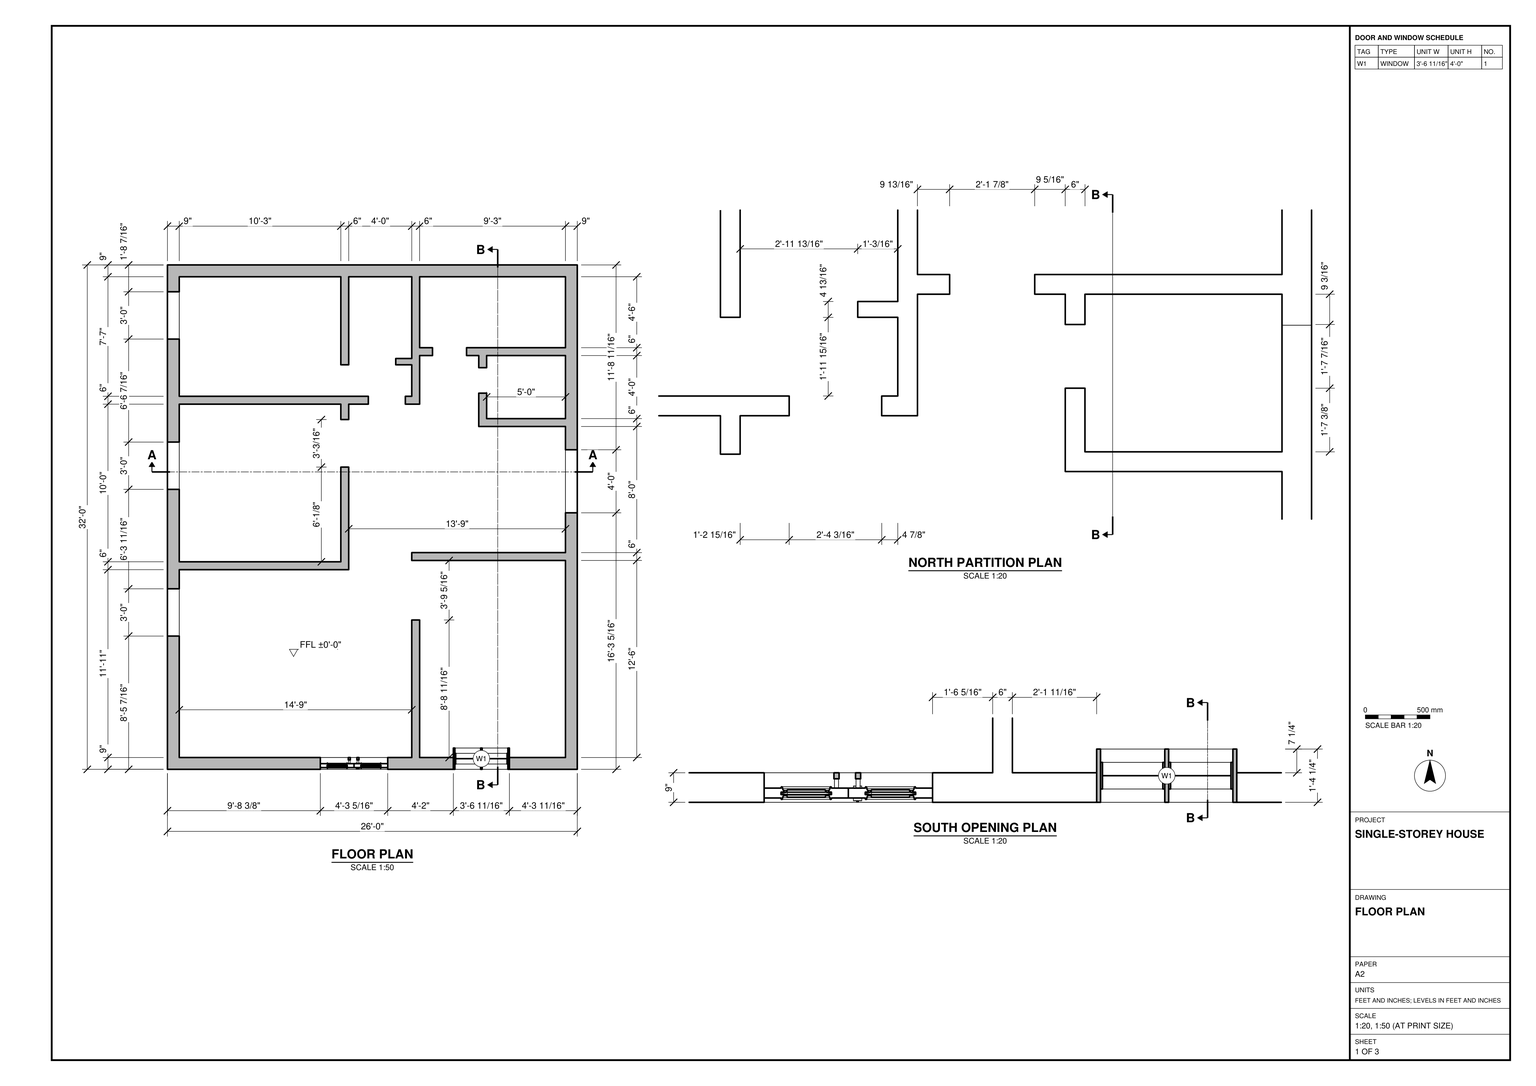
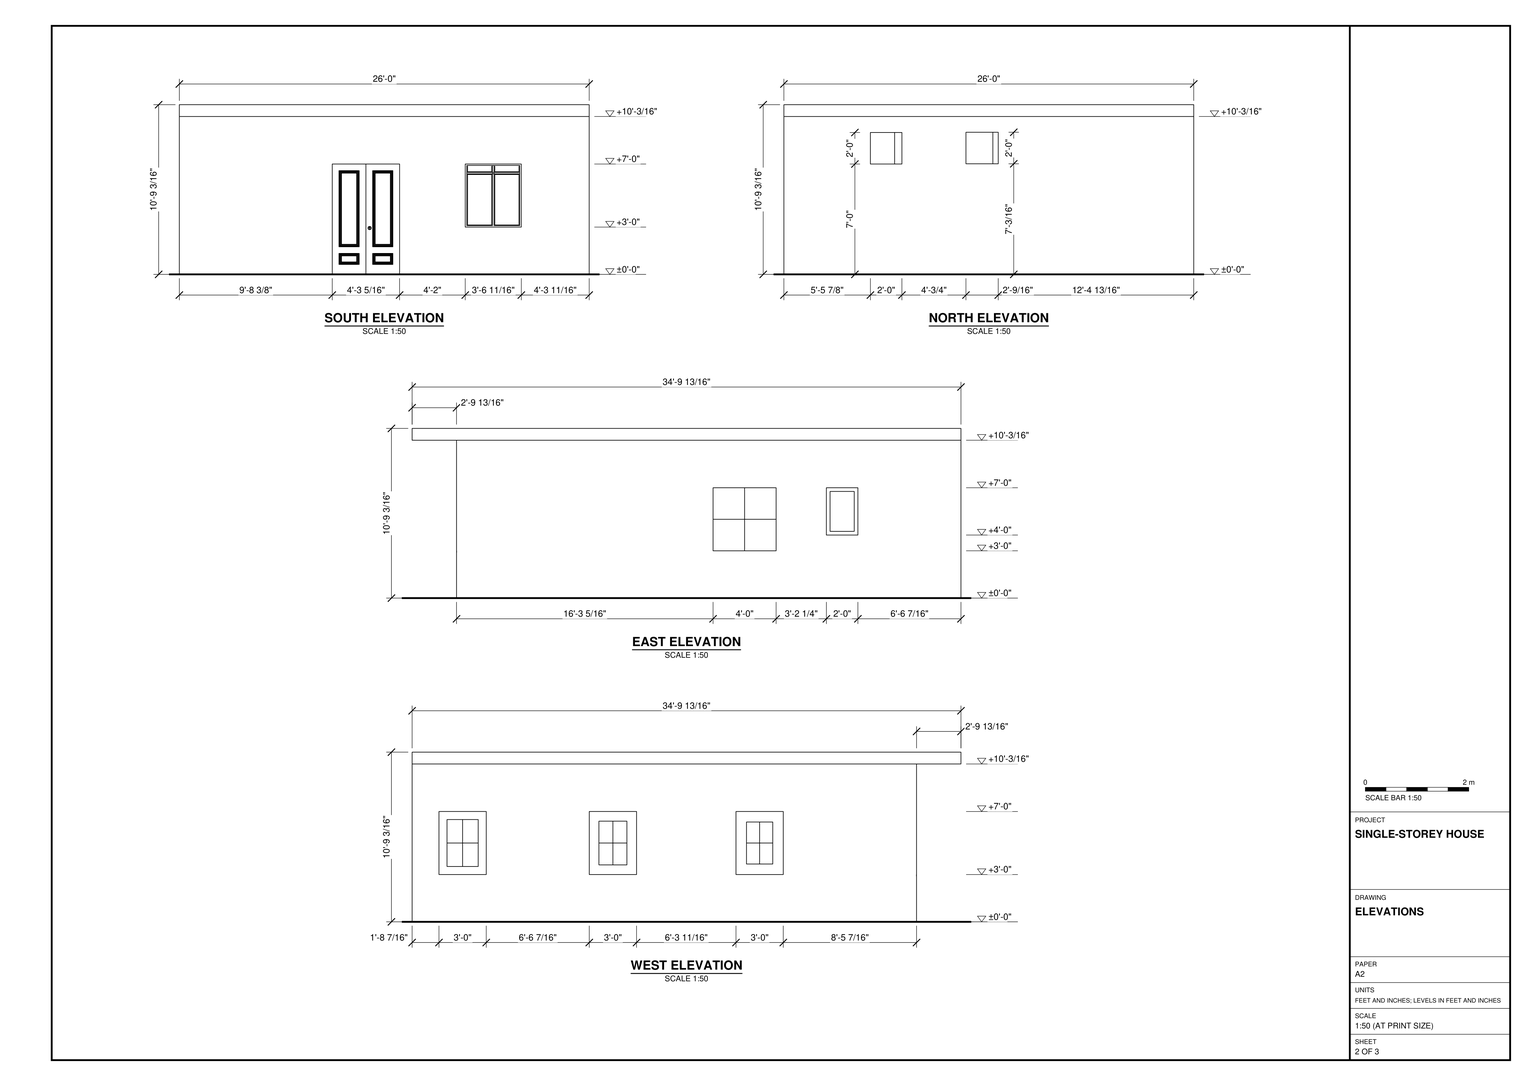
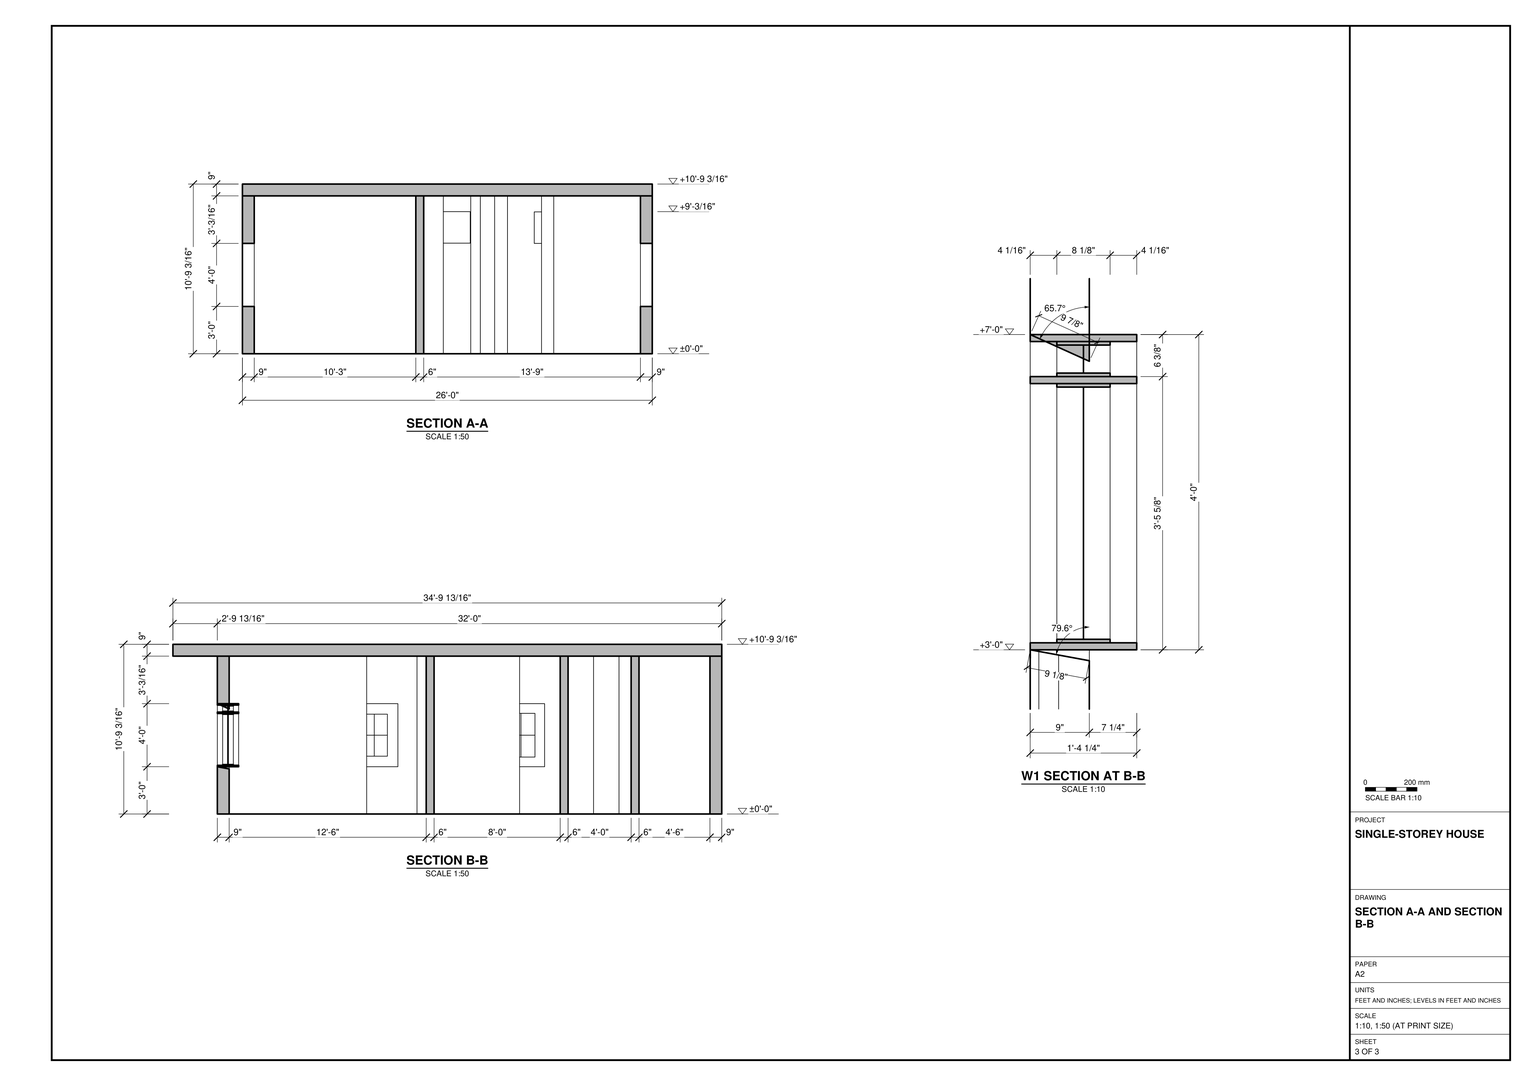
Build the single-storey house in SketchUp from task_files/diagram_01.pdf. Work in feet and inches. Set the finished ground floor at ±0'-0". The overall model is 26'-0" wide, 34'-9 13/16" deep and 10'-9 3/16" high. The wall footprint is only 32'-0" deep: the flat roof slab projects 2'-9 13/16" beyond the south entrance wall and finishes flush with the north wall.

Use the floor plan to lay out the 9" exterior walls and 6" interior partitions. Follow the enlarged north partition plan for the short returns and passage openings. Use section B-B to check the depths of the rooms from front to back. Model the paired entrance doors and the window to their right on the south elevation. Use the window section to shape its head and sill, and the elevation to place its central mullion and transom. Match the sizes, spacing and sill heights of the openings on the other three elevations.

Keep walls, slabs, the roof and each joinery or furniture piece as separate groups or components, and use components for repeated parts. Any decor or loose items may be suitable library components. Save one SketchUp model as output_files/single_storey_house_with_a_projecting_flat_roof.skp.

# SketchUp Ruby script. Lengths in inches.
U = 1.inch
M = Sketchup.active_model
def pt(a) = Geom::Point3d.new(a.map { |v| v * U })
def face(e, loops, mat)
  f = e.add_face(loops[0].map { |a| pt(a) })
  loops[1..].each { |l| e.add_face(l.map { |a| pt(a) }).erase! }
  f.material = f.back_material = mat if mat
  f
end
# faces: each face lists its corners as indices into pts; further lists are holes
def faces(e, pts, list, mat = nil) = list.each { |f| face(e, (f[0].is_a?(Array) ? f : [f]).map { |l| l.map { |i| pts[i] } }, mat) }
# xy, xz, yz: faces in a plane at the given z, y or x. An outline is a flat list of corners, or four numbers for a rectangle; further outlines are holes
def ring(l) = l.size == 4 ? [[l[0], l[1]], [l[2], l[1]], [l[2], l[3]], [l[0], l[3]]] : l.each_slice(2).to_a
def flat(e, list, mat, &to3) = list.each { |f| face(e, (f[0].is_a?(Array) ? f : [f]).map { |l| ring(l).map { |u, v| to3.(u, v) } }, mat) }
def xy(e, z, list, mat = nil) = flat(e, list, mat) { |x, y| [x, y, z] }
def xz(e, y, list, mat = nil) = flat(e, list, mat) { |x, z| [x, y, z] }
def yz(e, x, list, mat = nil) = flat(e, list, mat) { |y, z| [x, y, z] }
def lines(e, pts, list) = list.each { |a, b| e.add_line(pt(pts[a]), pt(pts[b])) }
# prism: a flat outline (further loops are holes) pulled along v
def prism(e, loops, v, mat = nil)
  f = face(e, loops, mat); d = Geom::Vector3d.new(v.map { |x| x * U })
  f.pushpull(f.normal.samedirection?(d) ? d.length : -d.length)
end
def box(e, o, s, mat = nil) = prism(e, [[o, [o[0] + s[0], o[1], o[2]], [o[0] + s[0], o[1] + s[1], o[2]], [o[0], o[1] + s[1], o[2]]]], [0, 0, s[2]], mat)
def at(x, y, z, deg = 0) = Geom::Transformation.translation(pt([x, y, z])) * Geom::Transformation.rotation(ORIGIN, Z_AXIS, deg.degrees)
def axes(o, x, y, z) = Geom::Transformation.new([*x, 0, *y, 0, *z, 0, *pt(o).to_a, 1])
def part(name) = M.definitions.add(name)
# library, detail: a bought-in or finely detailed component or shape, given as its bounding box
def library(name, o, s) = part(name).tap { |d| box(d.entities, o, s) }
def detail(e, o, s) = box(e.add_group.entities, o, s)
def put(e, d, t, mat = nil) = e.add_instance(d, t).tap { |i| i.material = mat if mat }
def group(e, t, mat = nil) = e.add_group.tap { |g| g.transformation = t; g.material = mat if mat }.entities
root = M.entities
M.materials.add("[Color A01]").color = [255, 204, 204]
M.materials.add("[Color A03]").color = [255, 101, 101]
M.materials.add("[Color B03]").color = [255, 140, 101]
M.materials.add("[Color C02]").color = [255, 204, 153]
M.materials.add("[Color D06]").color = [204, 153, 0]
M.materials.add("[Concrete Block Layers]").color = [147, 139, 140]
M.materials.add("[Formica Speckled Grey]").color = [94, 105, 111]
M.materials.add("[Translucent Glass Blue]").color = [100, 149, 237]
M.materials["[Translucent Glass Blue]"].alpha = 0.5
M.materials.add("[Translucent Glass Gray]").color = [128, 128, 128]
M.materials["[Translucent Glass Gray]"].alpha = 0.5
M.materials.add("[Translucent Glass Tinted]").color = [8, 201, 241]
M.materials["[Translucent Glass Tinted]"].alpha = 0.48
M.materials.add("[Water Dark Blue]").color = [21, 144, 187]
M.materials.add("[Wood Bamboo]").color = [177, 105, 43]
c1 = part("Group\#3")
xy(c1.entities,0,[[0,0,32.48,1.97]])
xy(c1.entities,0.98,[[0.98,0,31.5,0.98],[0.98,0.98,31.5,1.97]])
xy(c1.entities,8.86,[[0.98,0,31.5,0.98],[0.98,0.98,31.5,1.97]])
xy(c1.entities,9.84,[[0,0,32.48,1.97]])
xz(c1.entities,0,[[[0,0,32.48,9.84],[0.98,0.98,31.5,8.86]]])
xz(c1.entities,0.98,[[0.98,0.98,31.5,8.86]],"[Translucent Glass Gray]")
xz(c1.entities,1.97,[[[0,0,32.48,9.84],[0.98,0.98,31.5,8.86]]])
yz(c1.entities,0,[[0,0,1.97,9.84]])
yz(c1.entities,0.98,[[0,0.98,0.98,8.86],[0.98,0.98,1.97,8.86]])
yz(c1.entities,31.5,[[0,0.98,0.98,8.86],[0.98,0.98,1.97,8.86]])
yz(c1.entities,32.48,[[0,0,1.97,9.84]])
c2 = part("Group\#4")
xy(c2.entities,0,[[0,0,32.48,1.97]])
xy(c2.entities,0.98,[[0.98,0,31.5,0.98],[0.98,0.98,31.5,1.97]])
xy(c2.entities,71.85,[[0.98,0,31.5,0.98],[0.98,0.98,31.5,1.97]])
xy(c2.entities,72.83,[[0,0,32.48,1.97]])
xz(c2.entities,0,[[[0,0,32.48,72.83],[0.98,0.98,31.5,71.85]]])
xz(c2.entities,0.98,[[0.98,0.98,31.5,71.85]],"[Translucent Glass Gray]")
xz(c2.entities,1.97,[[[0,0,32.48,72.83],[0.98,0.98,31.5,71.85]]])
yz(c2.entities,0,[[0,0,1.97,72.83]])
yz(c2.entities,0.98,[[0,0.98,0.98,71.85],[0.98,0.98,1.97,71.85]])
yz(c2.entities,31.5,[[0,0.98,0.98,71.85],[0.98,0.98,1.97,71.85]])
yz(c2.entities,32.48,[[0,0,1.97,72.83]])
c3 = part("FIXED+GLASS+WINDOW+WITH+TRANSOM")
g1 = group(c3.entities,at(0,0,0))
xy(g1,0,[[0,0,70.86,3.9375]])
xy(g1,1.97,[[1.97,0,34.45,0.98],[36.42,0,68.9,3.9375],[1.97,2.95,34.45,3.9375]])
xy(g1,86.61,[[1.97,0,34.45,3.9375],[34.45,0,36.42,3.9375],[36.42,0,68.9,3.9375]])
xy(g1,88.58,[[0,0,70.86,3.9375]])
xz(g1,0,[[[0,0,70.86,88.58],[1.97,1.97,34.45,86.61],[36.42,1.97,68.9,86.61]]])
xz(g1,3.9375,[[[0,0,70.86,88.58],[1.97,1.97,34.45,86.61],[36.42,1.97,68.9,86.61]]])
yz(g1,0,[[0,0,3.9375,88.58]])
yz(g1,1.97,[[0,1.97,3.9375,74.8],[0,76.77,3.9375,86.61]])
yz(g1,34.45,[[0,1.97,3.9375,86.61]])
yz(g1,36.42,[[0,1.97,3.9375,86.61]])
yz(g1,68.9,[[0,1.97,3.9375,86.61]])
yz(g1,70.86,[[0,0,3.9375,88.58]])
g2 = group(g1,at(1.97,0,74.8))
box(g2,[0,0,0],[66.93,3.9375,1.97])
put(g1,c1,at(1.97,0.98,76.77))
put(g1,c1,at(36.42,0.98,76.77))
put(g1,c2,at(1.97,0.98,1.97))
put(g1,c2,at(36.42,0.98,1.97))
c4 = library("DD LT 2",[0,0,0],[47.24,4.7,78.74])
xy(root,0,[[0,33.8125,0,135.26,9,135.26,9,42.8125,116.41,42.8125,116.41,33.8125],[116.41,33.8125,167.6875,42.8125],[167.6875,33.8125,167.6875,42.8125,186,42.8125,186,147.5,192,147.5,192,42.8125,217.66,42.8125,217.66,33.8125],[217.66,33.8125,217.66,42.8125,303,42.8125,303,192.8125,186,192.8125,186,198.8125,303,198.8125,303,277.1,312,277.1,312,33.8125],[0,135.26,0,246.95,9,246.95,9,191.8125,132,191.8125,132,263.91,138,263.91,138,185.8125,9,185.8125,9,135.26],
  [0,246.95,0,361.37,9,361.37,9,317.8125,152.9375,317.8125,152.9375,311.8125,138,311.8125,138,300.1,132,300.1,132,311.8125,9,311.8125,9,246.95],[303,277.1,303,294.8125,237,294.8125,237,320.2,243,320.2,243,300.8125,303,300.8125,303,339.36,312,339.36,312,277.1],[181.1,311.8125,181.1,317.8125,186,317.8125,186,341.78,173.8125,341.78,173.8125,346.59,186,346.59,186,408.8125,173.41,408.8125,173.41,417.8125,222.16,417.8125,222.16,408.8125,192,408.8125,192,354.8125,201.79,354.8125,201.79,348.8125,192,348.8125,192,311.8125],[303,339.36,303,348.8125,243,348.8125,243,339.59,237,339.59,237,348.8125,227.7,348.8125,227.7,354.8125,303,354.8125,303,408.8125,222.16,408.8125,222.16,417.8125,312,417.8125,312,339.36],[132,341.78,132,408.8125,9,408.8125,9,361.37,0,361.37,0,417.8125,148.83,417.8125,148.83,408.8125,138,408.8125,138,341.78],
  [148.83,408.8125,173.41,417.8125]])
xy(root,0,[[9,42.8125,186,42.8125,186,147.5,192,147.5,192,42.8125,303,42.8125,303,192.8125,186,192.8125,186,198.8125,303,198.8125,303,294.8125,237,294.8125,237,320.2,243,320.2,243,300.8125,303,300.8125,303,348.8125,243,348.8125,243,339.59,237,339.59,237,348.8125,227.7,348.8125,227.7,354.8125,303,354.8125,303,408.8125,192,408.8125,192,354.8125,201.79,354.8125,201.79,348.8125,192,348.8125,192,311.8125,181.1,311.8125,181.1,317.8125,186,317.8125,186,341.78,173.8125,341.78,173.8125,346.59,186,346.59,186,408.8125,138,408.8125,138,341.78,132,341.78,132,408.8125,9,408.8125,9,317.8125,152.9375,317.8125,152.9375,311.8125,138,311.8125,138,300.1,132,300.1,132,311.8125,9,311.8125,9,191.8125,132,191.8125,132,263.91,138,263.91,138,185.8125,9,185.8125]],"[Wood Bamboo]")
xy(root,0.1875,[[181.1,311.8125,181.1,317.8125,186,317.8125,186,341.78,173.8125,341.78,173.8125,346.59,186,346.59,186,408.8125,173.41,408.8125,173.41,417.8125,222.16,417.8125,222.16,408.8125,192,408.8125,192,354.8125,201.79,354.8125,201.79,348.8125,192,348.8125,192,311.8125],[148.83,408.8125,173.41,417.8125]])
xy(root,36,[[0,135.26,9,171.26],[303,229.1,312,277.1],[0,246.95,9,282.95],[0,361.37,9,397.37]])
xy(root,48,[[303,315.36,312,339.36]])
xy(root,84,[[116.41,33.8125,167.6875,42.8125],[0,135.26,9,171.26],[303,229.1,312,277.1],[0,246.95,9,282.95],[303,315.36,312,339.36],
  [0,361.37,9,397.37],[222.16,408.8125,246.16,417.8125]])
xy(root,84.1875,[[148.83,408.8125,173.41,417.8125]])
xy(root,108,[[222.16,408.8125,246.16,417.8125]])
xy(root,108.1875,[[148.83,408.8125,173.41,417.8125]])
xy(root,120.1875,[[[0,33.8125,312,417.8125],[9,42.8125,9,185.8125,138,185.8125,138,263.91,132,263.91,132,191.8125,9,191.8125,9,311.8125,132,311.8125,132,300.1,138,300.1,138,311.8125,152.9375,311.8125,152.9375,317.8125,9,317.8125,9,408.8125,132,408.8125,132,341.78,138,341.78,138,408.8125,186,408.8125,186,346.59,173.8125,346.59,173.8125,341.78,186,341.78,186,317.8125,181.1,317.8125,181.1,311.8125,192,311.8125,192,348.8125,201.79,348.8125,201.79,354.8125,192,354.8125,192,408.8125,303,408.8125,303,354.8125,227.7,354.8125,227.7,348.8125,237,348.8125,237,339.59,243,339.59,243,348.8125,303,348.8125,303,300.8125,243,300.8125,243,320.2,237,320.2,237,294.8125,303,294.8125,303,198.8125,186,198.8125,186,192.8125,303,192.8125,303,42.8125,192,42.8125,192,147.5,186,147.5,186,42.8125]]],"[Color C02]")
xz(root,33.8125,[[[0,0,116.41,0,116.41,84,167.6875,84,167.6875,0,312,0,312,120.1875,0,120.1875],[217.66,36,260.33,84]]],"[Concrete Block Layers]")
xz(root,42.8125,[[9,0,9,120.1875,186,120.1875,186,0,167.6875,0,167.6875,84,116.41,84,116.41,0]],"[Color A03]")
xz(root,42.8125,[[[192,0,303,120.1875],[217.66,34.34,260.33,79.93]]],"[Color B03]")
xz(root,135.26,[[0,36,9,84]])
xz(root,147.5,[[186,0,192,120.1875]])
xz(root,171.26,[[0,36,9,84]])
xz(root,185.8125,[[9,0,138,120.1875]],"[Color A03]")
xz(root,191.8125,[[9,0,132,120.1875]],"[Color A01]")
xz(root,192.8125,[[186,0,192,120.1875],[192,0,303,120.1875]],"[Color B03]")
xz(root,198.8125,[[186,0,303,120.1875]],"[Formica Speckled Grey]")
xz(root,229.1,[[303,36,312,84]])
xz(root,246.95,[[0,36,9,84]])
xz(root,263.91,[[132,0,138,120.1875]])
xz(root,277.1,[[303,36,312,84]])
xz(root,282.95,[[0,36,9,84]])
xz(root,294.8125,[[237,0,303,120.1875]],"[Formica Speckled Grey]")
xz(root,300.1,[[132,0,138,120.1875]])
xz(root,300.8125,[[243,0,303,120.1875]],"[Formica Speckled Grey]")
xz(root,311.8125,[[181.1,0,192,0.1875]])
xz(root,311.8125,[[9,0,132,120.1875]],"[Color A01]")
xz(root,311.8125,[[138,0,152.9375,120.1875],[181.1,0.1875,192,120.1875]],"[Color C02]")
xz(root,315.36,[[303,48,312,84]])
xz(root,317.8125,[[181.1,0,186,0.1875],[181.1,0.1875,186,120.1875]])
xz(root,317.8125,[[9,0,152.9375,120.1875]],"[Color D06]")
xz(root,320.2,[[237,0,243,120.1875]])
xz(root,339.36,[[303,48,312,84]])
xz(root,339.59,[[237,0,243,120.1875]],"[Color A01]")
xz(root,341.78,[[132,0,138,120.1875],[173.8125,0,186,0.1875]])
xz(root,341.78,[[173.8125,0.1875,186,120.1875]],"[Color C02]")
xz(root,346.59,[[173.8125,0,186,0.1875]])
xz(root,346.59,[[173.8125,0.1875,186,120.1875]],"[Water Dark Blue]")
xz(root,348.8125,[[192,0,201.79,0.1875]])
xz(root,348.8125,[[227.7,0,237,120.1875]],"[Color A01]")
xz(root,348.8125,[[192,0.1875,201.79,120.1875]],"[Color C02]")
xz(root,348.8125,[[243,0,303,120.1875]],"[Formica Speckled Grey]")
xz(root,354.8125,[[192,0,201.79,0.1875]])
xz(root,354.8125,[[227.7,0,303,120.1875],[192,0.1875,201.79,120.1875]],"[Water Dark Blue]")
xz(root,361.37,[[0,36,9,84]])
xz(root,397.37,[[0,36,9,84]])
xz(root,408.8125,[[173.41,0,186,0.1875],[192,0,222.16,0.1875]])
xz(root,408.8125,[[9,0,132,120.1875]],"[Color D06]")
xz(root,408.8125,[[[138,0,148.83,0,148.83,0.1875,186,0.1875,186,120.1875,138,120.1875],[148.83,84.1875,173.41,108.1875]],[[222.16,0,303,0,303,120.1875,192,120.1875,192,0.1875,222.16,0.1875],[222.16,84,246.16,108]]],"[Water Dark Blue]")
xz(root,417.8125,[[173.41,0,222.16,0.1875]])
xz(root,417.8125,[[[0,0,0,120.1875,312,120.1875,312,0,222.16,0,222.16,0.1875,148.83,0.1875,148.83,0],[148.83,84.1875,173.41,108.1875],[222.16,84,246.16,108]]],"[Concrete Block Layers]")
yz(root,0,[[[135.26,36,171.26,84],[143.27,44.01,163.26,75.99]],[[246.95,36,282.95,84],[254.3,43.35,275.6,76.65]],[[361.37,36,397.37,84],[367.5,42.13,391.24,77.87]]])
yz(root,0,[[[33.8125,0,417.8125,120.1875],[135.26,36,171.26,84],[246.95,36,282.95,84],[361.37,36,397.37,84]]],"[Concrete Block Layers]")
yz(root,0,[[367.5,42.13,379.37,60],[379.37,42.13,391.24,60],[254.3,43.35,264.95,60],[264.95,43.35,275.6,60],[143.27,44.01,153.26,60],
  [153.26,44.01,163.26,60],[143.27,60,153.26,75.99],[153.26,60,163.26,75.99],[254.3,60,264.95,76.65],[264.95,60,275.6,76.65],
  [367.5,60,379.37,77.87],[379.37,60,391.24,77.87]],"[Translucent Glass Tinted]")
yz(root,9,[[[191.8125,0,311.8125,120.1875],[246.95,36,282.95,84]]],"[Color A01]")
yz(root,9,[[[42.8125,0,185.8125,120.1875],[135.26,36,171.26,84]]],"[Color A03]")
yz(root,9,[[[317.8125,0,408.8125,120.1875],[361.37,36,397.37,84]]],"[Color D06]")
yz(root,116.41,[[33.8125,0,42.8125,84]])
yz(root,132,[[191.8125,0,263.91,120.1875],[300.1,0,311.8125,120.1875]],"[Color A01]")
yz(root,132,[[341.78,0,408.8125,120.1875]],"[Color D06]")
yz(root,138,[[300.1,0,311.8125,120.1875]])
yz(root,138,[[185.8125,0,263.91,120.1875]],"[Color A01]")
yz(root,138,[[341.78,0,408.8125,120.1875]],"[Water Dark Blue]")
yz(root,148.83,[[408.8125,0,417.8125,0.1875],[408.8125,84.1875,417.8125,108.1875]])
yz(root,152.9375,[[311.8125,0,317.8125,120.1875]])
yz(root,167.6875,[[33.8125,0,42.8125,84]])
yz(root,173.41,[[408.8125,0,417.8125,0.1875],[408.8125,84.1875,417.8125,108.1875]])
yz(root,173.8125,[[341.78,0,346.59,0.1875],[341.78,0.1875,346.59,120.1875]])
yz(root,181.1,[[311.8125,0,317.8125,0.1875],[311.8125,0.1875,317.8125,120.1875]])
yz(root,186,[[192.8125,0,198.8125,120.1875],[317.8125,0,341.78,0.1875],[346.59,0,408.8125,0.1875],[317.8125,0.1875,341.78,120.1875]])
yz(root,186,[[42.8125,0,147.5,120.1875]],"[Color A03]")
yz(root,186,[[346.59,0.1875,408.8125,120.1875]],"[Water Dark Blue]")
yz(root,192,[[311.8125,0,348.8125,0.1875],[354.8125,0,408.8125,0.1875]])
yz(root,192,[[42.8125,0,147.5,120.1875]],"[Color B03]")
yz(root,192,[[311.8125,0.1875,348.8125,120.1875]],"[Color C02]")
yz(root,192,[[354.8125,0.1875,408.8125,120.1875]],"[Water Dark Blue]")
yz(root,201.79,[[348.8125,0,354.8125,0.1875]])
yz(root,201.79,[[348.8125,0.1875,354.8125,120.1875]],"[Color C02]")
yz(root,217.66,[[42.8125,34.34,42.8125,79.93,33.8125,84,33.8125,36]])
yz(root,222.16,[[408.8125,0,417.8125,0.1875],[408.8125,84,417.8125,108]])
yz(root,227.7,[[348.8125,0,354.8125,120.1875]])
yz(root,237,[[294.8125,0,320.2,120.1875],[339.59,0,348.8125,120.1875]],"[Formica Speckled Grey]")
yz(root,243,[[300.8125,0,320.2,120.1875],[339.59,0,348.8125,120.1875]],"[Formica Speckled Grey]")
yz(root,246.16,[[408.8125,84,417.8125,108]])
yz(root,260.33,[[42.8125,34.34,33.8125,36,33.8125,84,42.8125,79.93]])
yz(root,303,[[42.8125,0,192.8125,120.1875]],"[Color B03]")
yz(root,303,[[[198.8125,0,294.8125,120.1875],[229.1,36,277.1,84]],[[300.8125,0,348.8125,120.1875],[315.36,48,339.36,84]]],"[Formica Speckled Grey]")
yz(root,303,[[354.8125,0,408.8125,120.1875]],"[Water Dark Blue]")
yz(root,312,[[[315.36,48,339.36,84],[318.16,50.8,336.5625,81.2]]])
yz(root,312,[[[33.8125,0,417.8125,120.1875],[229.1,36,277.1,84],[315.36,48,339.36,84]]],"[Concrete Block Layers]")
yz(root,312,[[318.16,50.8,336.5625,81.2]],"[Translucent Glass Blue]")
yz(root,312,[[229.1,36,253.1,60],[253.1,36,277.1,60],[229.1,60,253.1,84],[253.1,60,277.1,84]],"[Translucent Glass Tinted]")
p = [[260.33,33.8125,36],[260.33,42.8125,34.34],[217.66,42.8125,34.34],[217.66,33.8125,36],[260.33,42.8125,79.93],[260.33,33.8125,84],
  [217.66,33.8125,84],[217.66,42.8125,79.93]]
faces(root,p,[[0,1,2,3],[4,5,6,7]])
put(root,c3,axes([217.66,50.03,36],[0.60216,0,0],[0,-4.12,0],[0,0,0.54187]))
put(root,c4,axes([116.41,42.8125,0],[1.08547,0,0],[0,-1.91297,0],[0,0,1.0668]))
g3 = group(root,at(0,33.8125,120.1875),"[Formica Speckled Grey]")
g4 = group(g3,at(0,-33.8125,0))
box(g4,[0,0,0],[312,417.8125,9])
